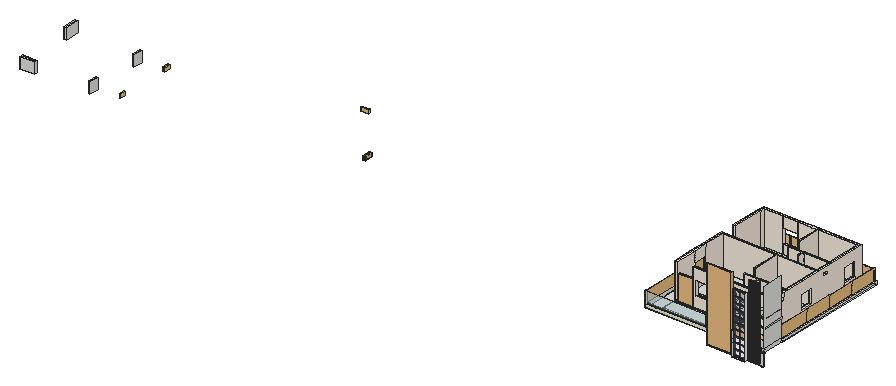
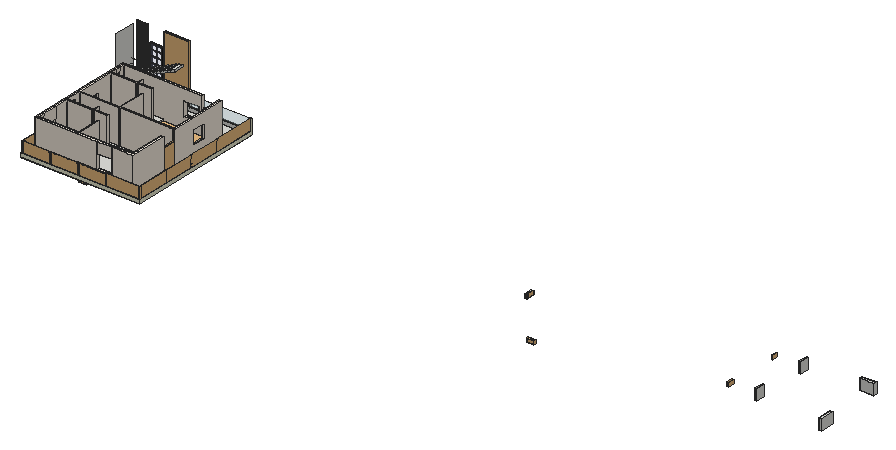
# SketchUp Ruby script. Lengths in inches.
U = 1.inch
M = Sketchup.active_model
def pt(a) = Geom::Point3d.new(a.map { |v| v * U })
def face(e, loops, mat)
  f = e.add_face(loops[0].map { |a| pt(a) })
  loops[1..].each { |l| e.add_face(l.map { |a| pt(a) }).erase! }
  f.material = f.back_material = mat if mat
  f
end
# faces: each face lists its corners as indices into pts; further lists are holes
def faces(e, pts, list, mat = nil) = list.each { |f| face(e, (f[0].is_a?(Array) ? f : [f]).map { |l| l.map { |i| pts[i] } }, mat) }
# xy, xz, yz: faces in a plane at the given z, y or x. An outline is a flat list of corners, or four numbers for a rectangle; further outlines are holes
def ring(l) = l.size == 4 ? [[l[0], l[1]], [l[2], l[1]], [l[2], l[3]], [l[0], l[3]]] : l.each_slice(2).to_a
def flat(e, list, mat, &to3) = list.each { |f| face(e, (f[0].is_a?(Array) ? f : [f]).map { |l| ring(l).map { |u, v| to3.(u, v) } }, mat) }
def xy(e, z, list, mat = nil) = flat(e, list, mat) { |x, y| [x, y, z] }
def xz(e, y, list, mat = nil) = flat(e, list, mat) { |x, z| [x, y, z] }
def yz(e, x, list, mat = nil) = flat(e, list, mat) { |y, z| [x, y, z] }
def lines(e, pts, list) = list.each { |a, b| e.add_line(pt(pts[a]), pt(pts[b])) }
# prism: a flat outline (further loops are holes) pulled along v
def prism(e, loops, v, mat = nil)
  f = face(e, loops, mat); d = Geom::Vector3d.new(v.map { |x| x * U })
  f.pushpull(f.normal.samedirection?(d) ? d.length : -d.length)
end
def box(e, o, s, mat = nil) = prism(e, [[o, [o[0] + s[0], o[1], o[2]], [o[0] + s[0], o[1] + s[1], o[2]], [o[0], o[1] + s[1], o[2]]]], [0, 0, s[2]], mat)
def at(x, y, z, deg = 0) = Geom::Transformation.translation(pt([x, y, z])) * Geom::Transformation.rotation(ORIGIN, Z_AXIS, deg.degrees)
def axes(o, x, y, z) = Geom::Transformation.new([*x, 0, *y, 0, *z, 0, *pt(o).to_a, 1])
def part(name) = M.definitions.add(name)
# library, detail: a bought-in or finely detailed component or shape, given as its bounding box
def library(name, o, s) = part(name).tap { |d| box(d.entities, o, s) }
def detail(e, o, s) = box(e.add_group.entities, o, s)
def put(e, d, t, mat = nil) = e.add_instance(d, t).tap { |i| i.material = mat if mat }
def group(e, t, mat = nil) = e.add_group.tap { |g| g.transformation = t; g.material = mat if mat }.entities
root = M.entities
M.materials.add("0037 AP 8028 PEACH ORGANZA").color = [246, 236, 223]
M.materials.add("0113 AP L161 ABSOLUTE WHITE").color = [243, 242, 236]
M.materials.add("0746 AP 7715 LUMINOUS").color = [235, 235, 209]
M.materials.add("Glass_Safety_01").color = [204, 235, 244]
M.materials["Glass_Safety_01"].alpha = 0.25
M.materials.add("Glass_Sky Reflection_01").color = [126, 138, 183]
M.materials["Glass_Sky Reflection_01"].alpha = 0.25
M.materials.add("M08_Obsidian_Black").color = [30, 30, 30]
M.materials.add("[0132_LightGray]").color = [169, 169, 169]
M.materials.add("[Metal Seamed]").color = [118, 119, 114]
c1 = library("Group\#46",[0,-3,0],[81.91,6,241.7])
c2 = library("Group\#25",[0,-0.05,0],[30,2.55,24])
c3 = part("Group19\#1")
p = [[1706.5625,247.76,0],[1706.5625,271.76,0],[1706.5625,427.76,65],[1706.5625,431.76,65],[1720.5625,431.76,65],[1720.5625,427.76,65],
  [1686.5625,247.76,0],[1686.5625,271.76,0],[1686.5625,427.76,65],[1686.5625,451.76,65],[1740.5625,451.76,65],[1740.5625,427.76,65]]
lines(c3.entities,p,[[0,1],[1,2],[2,3],[3,4],[4,5],[6,7],[7,8],[8,9],[9,10],[10,11]])
c4 = part("Group18\#2")
xy(c4.entities,-3.9375,[[1682.5625,269.14,1710.5625,281.14],[1684.29,281.14,1710.5625,281.93]])
xy(c4.entities,0,[[1682.5625,269.14,1710.5625,281.14]])
xy(c4.entities,5,[[1684.29,281.14,1710.5625,293.14]])
xy(c4.entities,10,[[1684.29,293.14,1710.5625,305.14]])
xy(c4.entities,15,[[1684.29,305.14,1710.5625,317.14]])
xy(c4.entities,20,[[1684.29,317.14,1710.5625,329.14]])
xy(c4.entities,25,[[1684.29,329.14,1710.5625,341.14]])
xy(c4.entities,30,[[1684.29,341.14,1710.5625,353.14]])
xy(c4.entities,35,[[1684.29,353.14,1710.5625,365.14]])
xy(c4.entities,40,[[1684.29,365.14,1710.5625,377.14]])
xy(c4.entities,45,[[1684.29,377.14,1710.5625,389.14]])
xy(c4.entities,50,[[1684.29,389.14,1710.5625,401.14]])
xy(c4.entities,55,[[1684.29,401.14,1710.5625,413.14]])
xy(c4.entities,60,[[1684.29,413.14,1710.5625,425.14]])
xy(c4.entities,61.0625,[[1716.5625,412.36,1744.5625,453.14],[1710.5625,425.14,1710.5625,437.93,1684.29,437.93,1684.29,453.14,1716.5625,453.14,1716.5625,425.14]])
xy(c4.entities,65,[[1716.5625,413.14,1744.5625,453.14],[1684.29,425.14,1716.5625,453.14]])
xy(c4.entities,70,[[1716.5625,401.14,1744.5625,413.14]])
xy(c4.entities,75,[[1716.5625,389.14,1744.5625,401.14]])
xy(c4.entities,80,[[1716.5625,377.14,1744.5625,389.14]])
xy(c4.entities,85,[[1716.5625,365.14,1744.5625,377.14]])
xy(c4.entities,90,[[1716.5625,353.14,1744.5625,365.14]])
xy(c4.entities,95,[[1716.5625,341.14,1744.5625,353.14]])
xy(c4.entities,100,[[1716.5625,329.14,1744.5625,341.14]])
xy(c4.entities,105,[[1716.5625,317.14,1744.5625,329.14]])
xy(c4.entities,110,[[1716.5625,305.14,1744.5625,317.14]])
xy(c4.entities,115,[[1716.5625,293.14,1744.5625,305.14]])
xy(c4.entities,120.6,[[1716.5625,281.14,1744.5625,293.14]])
xz(c4.entities,269.14,[[1682.5625,-3.9375,1710.5625,0]])
xz(c4.entities,281.14,[[1682.5625,-3.9375,1684.29,0],[1684.29,-3.9375,1710.5625,0],[1684.29,0,1710.5625,5],[1716.5625,115.73,1744.5625,120.6]])
xz(c4.entities,293.14,[[1684.29,5,1710.5625,10],[1716.5625,115,1744.5625,120.6]])
xz(c4.entities,305.14,[[1684.29,10,1710.5625,15],[1716.5625,110,1744.5625,115]])
xz(c4.entities,317.14,[[1684.29,15,1710.5625,20],[1716.5625,105,1744.5625,110]])
xz(c4.entities,329.14,[[1684.29,20,1710.5625,25],[1716.5625,100,1744.5625,105]])
xz(c4.entities,341.14,[[1684.29,25,1710.5625,30],[1716.5625,95,1744.5625,100]])
xz(c4.entities,353.14,[[1684.29,30,1710.5625,35],[1716.5625,90,1744.5625,95]])
xz(c4.entities,365.14,[[1684.29,35,1710.5625,40],[1716.5625,85,1744.5625,90]])
xz(c4.entities,377.14,[[1684.29,40,1710.5625,45],[1716.5625,80,1744.5625,85]])
xz(c4.entities,389.14,[[1684.29,45,1710.5625,50],[1716.5625,75,1744.5625,80]])
xz(c4.entities,401.14,[[1684.29,50,1710.5625,55],[1716.5625,70,1744.5625,75]])
xz(c4.entities,413.14,[[1684.29,55,1710.5625,60],[1716.5625,65,1744.5625,70]])
xz(c4.entities,425.14,[[1684.29,60,1710.5625,65],[1710.5625,61.0625,1716.5625,65]])
xz(c4.entities,453.14,[[1684.29,61.0625,1716.5625,65],[1716.5625,61.0625,1744.5625,65]])
yz(c4.entities,1682.5625,[[269.14,-3.9375,281.14,0]])
yz(c4.entities,1684.29,[[281.14,-3.9375,281.14,5,293.14,5,293.14,10,305.14,10,305.14,15,317.14,15,317.14,20,329.14,20,329.14,25,341.14,25,341.14,30,353.14,30,353.14,35,365.14,35,365.14,40,377.14,40,377.14,45,389.14,45,389.14,50,401.14,50,401.14,55,413.14,55,413.14,60,425.14,60,425.14,65,453.14,65,453.14,61.0625,437.93,61.0625,281.93,-3.9375]])
yz(c4.entities,1710.5625,[[269.14,-3.9375,281.14,0],[281.14,-3.9375,281.93,-3.9375,437.93,61.0625,425.14,61.0625,425.14,60,413.14,60,413.14,55,401.14,55,401.14,50,389.14,50,389.14,45,377.14,45,377.14,40,365.14,40,365.14,35,353.14,35,353.14,30,341.14,30,341.14,25,329.14,25,329.14,20,317.14,20,317.14,15,305.14,15,305.14,10,293.14,10,293.14,5,281.14,5]])
yz(c4.entities,1716.5625,[[412.36,61.0625,281.42,115.62,281.14,115.73,281.14,120.6,293.14,120.6,293.14,115,305.14,115,305.14,110,317.14,110,317.14,105,329.14,105,329.14,100,341.14,100,341.14,95,353.14,95,353.14,90,365.14,90,365.14,85,377.14,85,377.14,80,389.14,80,389.14,75,401.14,75,401.14,70,413.14,70,413.14,65,425.14,65,425.14,61.0625],[425.14,61.0625,453.14,65]])
yz(c4.entities,1744.5625,[[412.36,61.0625,453.14,61.0625,453.14,65,413.14,65,413.14,70,401.14,70,401.14,75,389.14,75,389.14,80,377.14,80,377.14,85,365.14,85,365.14,90,353.14,90,353.14,95,341.14,95,341.14,100,329.14,100,329.14,105,317.14,105,317.14,110,305.14,110,305.14,115,293.14,115,293.14,120.6,281.14,120.6,281.14,115.73]])
p = [[1710.5625,281.93,-3.9375],[1684.29,281.93,-3.9375],[1684.29,437.93,61.0625],[1710.5625,437.93,61.0625],[1744.5625,412.36,61.0625],[1744.5625,281.14,115.73],
  [1716.5625,281.42,115.62],[1716.5625,412.36,61.0625],[1716.5625,281.14,115.73]]
faces(c4.entities,p,[[0,1,2,3],[4,5,6,7],[8,6,5]])
put(c4.entities,c3,at(0,0,24))
c5 = library("Group\#2",[41.39,24.57,0],[327.06,423.03,0.01])
c6 = library("Group\#12",[0,0,0],[6.9375,42,86.5])
c7 = part("Group\#29")
xy(c7.entities,0,[[0,0,0,179.49,176.02,179.49,176.02,89,180.99,89,180.99,179.49,311,179.49,311,53,176.02,53,176.02,47.99,222,47.99,222,30.01,227.01,30.01,227.01,47.99,311,47.99,311,0]])
c8 = library("skp9290",[5.02,1.95,0],[10.03,3.89,0.08])
box(root,[272,323.41,84],[5.01,30,36])
box(root,[272,138.91,84],[5.01,30,36])
box(root,[50,129.92,84],[48.03,8.99,36])
box(root,[41.01,323.41,84],[8.99,47.98,36])
xy(root,73.55,[[2370.2,117.37,2549.9,117.53]])
xy(root,73.55,[[2452.6,108.36,2495.6,117.37]],"0113 AP L161 ABSOLUTE WHITE")
xy(root,80.8,[[2370.2,103.36,2448.6,112.36],[2506.22,109.7,2507.72,110.7],[2511.22,109.7,2512.72,110.7],[2516.22,109.7,2517.72,110.7],[2521.22,109.7,2522.72,110.7],
  [2526.22,109.7,2527.72,110.7],[2531.22,109.7,2532.72,110.7],[2536.22,109.7,2537.72,110.7],[2541.22,109.7,2542.72,110.7],[2366.69,112.36,2370.2,117.37]])
xy(root,92.44,[[2519.38,354.52,2528.37,379.54]])
xy(root,96,[[1066.63,294.4,1075.625,319.41]])
xy(root,104.08,[[2519.38,354.52,2528.37,379.54]])
xy(root,108,[[1066.63,294.4,1075.625,319.41]])
xy(root,115.5,[[2155.9,112.36,2160.9,117.37],[2160.9,112.36,2366.69,117.37],[2549.9,112.36,2550.375,117.37],[2155.9,117.37,2160.9,579.4],[2549.9,117.37,2550.375,117.53],
  [2525.88,189.89,2549.9,192.78],[2549.9,192.78,2554.91,584.4],[2155.9,579.4,2549.9,584.4]])
xy(root,127.5,[[2160.9,112.36,2366.69,112.36,2366.69,117.37,2160.9,117.37,2160.9,115.67,2361.69,115.67,2361.69,113.67,2160.9,113.67],[2160.9,113.67,2361.69,115.67],[2155.9,117.37,2160.9,579.4],[2549.9,189.89,2554.91,584.4],[2155.9,579.4,2549.9,584.4]])
xz(root,109.7,[[2506.22,80.8,2507.72,322.5],[2511.22,80.8,2512.72,322.5],[2516.22,80.8,2517.72,322.5],[2521.22,80.8,2522.72,322.5],[2526.22,80.8,2527.72,322.5],
  [2531.22,80.8,2532.72,322.5],[2536.22,80.8,2537.72,322.5],[2541.22,80.8,2542.72,322.5]],"[0132_LightGray]")
xz(root,110.7,[[2506.22,80.8,2507.72,322.5],[2511.22,80.8,2512.72,322.5],[2516.22,80.8,2517.72,322.5],[2521.22,80.8,2522.72,322.5],[2526.22,80.8,2527.72,322.5],
  [2531.22,80.8,2532.72,322.5],[2536.22,80.8,2537.72,322.5],[2541.22,80.8,2542.72,322.5]])
xz(root,112.36,[[2155.9,115.5,2366.69,115.5,2366.69,127.5,2160.9,127.5,2160.9,164.58,2155.9,164.58]],"0746 AP 7715 LUMINOUS")
xz(root,113.67,[[2160.9,127.5,2361.69,164.58]],"Glass_Safety_01")
xz(root,115.67,[[2160.9,127.5,2361.69,164.58]],"Glass_Safety_01")
xz(root,117.37,[[2370.2,73.55,2452.6,115.5],[2495.6,73.55,2549.9,115.5],[2366.69,80.8,2370.2,115.5],[2160.9,115.5,2452.6,127.5],[2495.6,115.5,2549.9,127.5],
  [2366.69,127.5,2452.6,151.5],[2495.6,127.5,2549.9,151.5]])
xz(root,117.37,[[2155.9,127.5,2160.9,164.58]],"0746 AP 7715 LUMINOUS")
xz(root,294.4,[[1066.63,96,1075.625,108]])
xz(root,319.41,[[1066.63,96,1075.625,108]])
xz(root,354.52,[[2519.38,92.44,2528.37,104.08]])
xz(root,379.54,[[2519.38,92.44,2528.37,104.08]])
xz(root,579.4,[[2160.9,115.5,2549.9,127.5]])
xz(root,584.4,[[2155.9,115.5,2554.91,127.5]],"0746 AP 7715 LUMINOUS")
yz(root,2155.9,[[112.36,115.5,112.36,164.58,117.37,164.58,117.37,127.5,584.4,127.5,584.4,115.5]],"0746 AP 7715 LUMINOUS")
yz(root,2160.9,[[117.37,115.5,579.4,127.5],[112.36,127.5,113.67,164.58],[113.67,127.5,115.67,164.58],[115.67,127.5,117.37,164.58]])
yz(root,2361.69,[[113.67,127.5,115.67,164.58]])
yz(root,2366.69,[[112.36,127.5,117.37,151.5]])
yz(root,2366.69,[[112.36,80.8,117.37,115.5]],"0746 AP 7715 LUMINOUS")
yz(root,2448.6,[[108.36,80.8,112.36,151.5]])
yz(root,2452.6,[[108.36,115.5,117.37,127.5],[108.36,127.5,117.37,151.49]])
yz(root,2452.6,[[108.36,73.55,117.37,115.5]],"0113 AP L161 ABSOLUTE WHITE")
yz(root,2495.6,[[108.36,73.55,117.37,274.5]],"0113 AP L161 ABSOLUTE WHITE")
yz(root,2506.22,[[109.7,80.8,110.7,322.5]],"[0132_LightGray]")
yz(root,2507.72,[[109.7,80.8,110.7,322.5]],"[0132_LightGray]")
yz(root,2511.22,[[109.7,80.8,110.7,322.5]],"[0132_LightGray]")
yz(root,2512.72,[[109.7,80.8,110.7,322.5]],"[0132_LightGray]")
yz(root,2516.22,[[109.7,80.8,110.7,322.5]],"[0132_LightGray]")
yz(root,2517.72,[[109.7,80.8,110.7,322.5]],"[0132_LightGray]")
yz(root,2521.22,[[109.7,80.8,110.7,322.5]],"[0132_LightGray]")
yz(root,2522.72,[[109.7,80.8,110.7,322.5]],"[0132_LightGray]")
yz(root,2525.88,[[189.89,115.5,192.78,235.5]])
yz(root,2526.22,[[109.7,80.8,110.7,322.5]],"[0132_LightGray]")
yz(root,2527.72,[[109.7,80.8,110.7,322.5]],"[0132_LightGray]")
yz(root,2531.22,[[109.7,80.8,110.7,322.5]],"[0132_LightGray]")
yz(root,2532.72,[[109.7,80.8,110.7,322.5]],"[0132_LightGray]")
yz(root,2536.22,[[109.7,80.8,110.7,322.5]],"[0132_LightGray]")
yz(root,2537.72,[[109.7,80.8,110.7,322.5]],"[0132_LightGray]")
yz(root,2541.22,[[109.7,80.8,110.7,322.5]],"[0132_LightGray]")
yz(root,2542.72,[[109.7,80.8,110.7,322.5]],"[0132_LightGray]")
yz(root,2549.9,[[117.37,73.55,117.53,115.5],[112.36,115.5,117.37,127.5],[117.37,115.5,579.4,127.5],[117.37,127.5,189.89,313.5]])
p = [[2528.375,194.04,120],[2554.91,194.04,120],[2554.91,112.36,120],[2550.375,112.36,120],[2550.375,191.07,120],[2554.91,191.07,120],
  [2554.91,189.89,115.5],[2549.9,189.89,115.5],[2549.9,117.37,127.5],[2554.91,117.37,127.5],[2550.375,112.36,115.5],[2554.91,112.36,115.5],
  [2550.375,117.37,115.5],[2554.91,117.37,115.5],[2370.2,112.36,115.5],[2370.2,117.37,115.5]]
lines(root,p,[[0,1],[2,3],[4,5],[6,7],[8,9],[10,11],[12,13],[14,15]])
g1 = group(root,at(2452.6,117.3,73.55),"M08_Obsidian_Black")
xy(g1,0,[[42.95,-4.93,-0.06,-4.2,0,0.73,43,0]])
xy(g1,0.8,[[41.96,-4.91,41.97,-3.72,21.66,-3.37,21.46,-3.37,0.94,-3.02,0.93,-4.22],[41.97,-3.72,42.01,0.02,0.99,0.71,0.94,-3.02,21.46,-3.37,21.66,-3.37]])
xy(g1,200.15,[[41.96,-4.91,0.93,-4.22,0.94,-3.02,21.46,-3.37,21.66,-3.37,41.97,-3.72],[41.97,-3.72,21.66,-3.37,21.46,-3.37,0.94,-3.02,0.99,0.71,42.01,0.02]])
xy(g1,200.95,[[42.95,-4.93,43,0,0,0.73,-0.06,-4.2]])
xz(g1,-3.37,[[21.46,0.8,21.66,200.15]],"M08_Obsidian_Black")
p = [[42.95,-4.93,200.95],[-0.06,-4.2,200.95],[-0.06,-4.2,0],[42.95,-4.93,0],[41.96,-4.91,0.8],[0.93,-4.22,0.8],
  [0.93,-4.22,200.15],[41.96,-4.91,200.15],[43,0,0],[43,0,200.95],[0,0.73,200.95],[0,0.73,0],
  [0.99,0.71,0.8],[42.01,0.02,0.8],[42.01,0.02,200.15],[0.99,0.71,200.15],[41.97,-3.72,200.15],[41.97,-3.72,199.98],
  [41.97,-3.72,180.28],[41.97,-3.72,180.11],[41.97,-3.72,160.41],[41.97,-3.72,160.24],[41.97,-3.72,140.54],[41.97,-3.72,140.37],
  [41.97,-3.72,120.67],[41.97,-3.72,120.5],[41.97,-3.72,100.8],[41.97,-3.72,100.63],[41.97,-3.72,80.93],[41.97,-3.72,80.76],
  [41.97,-3.72,61.06],[41.97,-3.72,60.89],[41.97,-3.72,41.19],[41.97,-3.72,41.02],[41.97,-3.72,21.32],[41.97,-3.72,21.15],
  [41.97,-3.72,1.45],[41.97,-3.72,1.28],[41.97,-3.72,0.8],[0.94,-3.02,0.8],[0.94,-3.02,1.28],[0.94,-3.02,1.45],
  [0.94,-3.02,21.15],[0.94,-3.02,21.32],[0.94,-3.02,41.02],[0.94,-3.02,41.19],[0.94,-3.02,60.89],[0.94,-3.02,61.06],
  [0.94,-3.02,80.76],[0.94,-3.02,80.93],[0.94,-3.02,100.63],[0.94,-3.02,100.8],[0.94,-3.02,120.5],[0.94,-3.02,120.67],
  [0.94,-3.02,140.37],[0.94,-3.02,140.54],[0.94,-3.02,160.24],[0.94,-3.02,160.41],[0.94,-3.02,180.11],[0.94,-3.02,180.28],
  [0.94,-3.02,199.98],[0.94,-3.02,200.15],[21.66,-3.37,1.28],[21.66,-3.37,0.8],[21.46,-3.37,0.8],[21.46,-3.37,1.28],
  [21.66,-3.37,1.45],[21.46,-3.37,1.45],[21.66,-3.37,21.15],[21.46,-3.37,21.15],[21.66,-3.37,21.32],[21.46,-3.37,21.32],
  [21.66,-3.37,41.02],[21.46,-3.37,41.02],[21.66,-3.37,41.19],[21.46,-3.37,41.19],[21.66,-3.37,60.89],[21.46,-3.37,60.89],
  [21.66,-3.37,61.06],[21.46,-3.37,61.06],[21.66,-3.37,80.76],[21.46,-3.37,80.76],[21.66,-3.37,80.93],[21.46,-3.37,80.93],
  [21.66,-3.37,100.63],[21.46,-3.37,100.63],[21.66,-3.37,100.8],[21.46,-3.37,100.8],[21.66,-3.37,120.5],[21.46,-3.37,120.5],
  [21.66,-3.37,120.67],[21.46,-3.37,120.67],[21.66,-3.37,140.37],[21.46,-3.37,140.37],[21.66,-3.37,140.54],[21.46,-3.37,140.54],
  [21.66,-3.37,160.24],[21.46,-3.37,160.24],[21.66,-3.37,160.41],[21.46,-3.37,160.41],[21.66,-3.37,180.11],[21.46,-3.37,180.11],
  [21.66,-3.37,180.28],[21.46,-3.37,180.28],[21.66,-3.37,199.98],[21.46,-3.37,199.98],[21.66,-3.37,200.15],[21.46,-3.37,200.15]]
faces(g1,p,[[[0,1,2,3],[4,5,6,7]],[66,62,37,36],[65,67,41,40],[70,68,35,34],[69,71,43,42],[74,72,33,32],[73,75,45,44],[78,76,31,30],
  [77,79,47,46],[82,80,29,28],[81,83,49,48],[86,84,27,26],[85,87,51,50],[90,88,25,24],[89,91,53,52],[94,92,23,22],
  [93,95,55,54],[98,96,21,20],[97,99,57,56],[102,100,19,18],[101,103,59,58],[106,104,17,16],[61,60,105,107]],"M08_Obsidian_Black")
faces(g1,p,[[8,9,0,3],[10,11,2,1],[[10,9,8,11],[12,13,14,15]],[7,16,17,18,19,20,21,22,23,24,25,26,27,28,29,30,31,32,33,34,35,36,37,38,4],[5,39,40,41,42,43,44,45,46,47,48,49,50,51,52,53,54,55,56,57,58,59,60,61,6],[14,13,38,37,36,35,34,33,32,31,30,29,28,27,26,25,24,23,22,21,20,19,18,17,16],[12,15,61,60,59,58,57,56,55,54,53,52,51,50,49,48,47,46,45,44,43,42,41,40,39]])
faces(g1,p,[[38,37,62,63],[64,65,40,39],[68,66,36,35],[42,41,67,69],[72,70,34,33],[44,43,71,73],[76,74,32,31],[46,45,75,77],
  [80,78,30,29],[48,47,79,81],[84,82,28,27],[50,49,83,85],[88,86,26,25],[52,51,87,89],[92,90,24,23],[54,53,91,93],
  [96,94,22,21],[56,55,95,97],[100,98,20,19],[58,57,99,101],[104,102,18,17],[60,59,103,105]],"Glass_Sky Reflection_01")
put(root,c1,at(2366.69,112.36,80.8))
put(root,c2,axes([2354.36,553.61,92.44],[0.8,0,0],[0,1.82683,0],[0,0,0.485]))
put(root,c2,axes([2521.38,379.54,92.44],[0,-0.83382,0],[1.82683,0,0],[0,0,0.485]))
put(root,c2,axes([363,171.91,95.92],[0,-0.60073,0],[1.82683,0,0],[0,0,0.50315]))
put(root,c2,axes([363,357.39,95.92],[0,-0.66205,0],[1.82683,0,0],[0,0,0.51171]))
put(root,c2,axes([901.62,493.49,96],[0.8,0,0],[0,1.82683,0],[0,0,0.5]))
put(root,c2,axes([1068.63,319.41,96],[0,-0.83382,0],[1.82683,0,0],[0,0,0.5]))
put(root,c4,axes([2084.98,2150.13,119.72],[0.0107,-1.16479,0],[0.99132,0.00911,0],[0,0,1.07141]))
g2 = group(root,at(2160.9,560.39,115.5))
xy(g2,0,[[0,-443.02,36,-370.5],[36,-443.02,209.22,-370.5],[0,-370.5,36,0],[209.22,-370.5,364.98,-367.61],[364.98,-367.61,388.99,0],
  [0,0,364.98,19.01],[364.98,0,388.99,19.01]])
xy(g2,1,[[0,-443.02,209.22,-443.02,209.22,-370.5,36,-370.5,36,0,364.98,0,364.98,19.01,0,19.01],[209.22,-370.5,364.98,-367.61],[364.98,-367.61,388.99,0],[364.98,0,388.99,19.01]])
xz(g2,-443.02,[[0,0,36,1],[36,0,209.22,1]])
xz(g2,-370.5,[[36,0,364.98,1]])
xz(g2,-367.61,[[209.22,0,388.99,1]])
xz(g2,0,[[36,0,364.98,1],[364.98,0,388.99,1]])
xz(g2,19.01,[[0,0,364.98,1],[364.98,0,388.99,1]])
yz(g2,0,[[-443.02,0,-370.5,1],[-370.5,0,0,1],[0,0,19.01,1]])
yz(g2,36,[[-370.5,0,0,1]])
yz(g2,209.22,[[-443.02,0,-367.61,1]])
yz(g2,364.98,[[-370.5,0,0,1],[0,0,19.01,1]])
yz(g2,388.99,[[-367.61,0,0,1],[0,0,19.01,1]])
put(root,c5,at(2155.9,112.36,115.5))
put(root,c6,axes([2426.9,383.38,115.5],[0.86547,0,0],[0,0.71448,0],[0,0,0.9711]))
put(root,c6,axes([2253.93,190.32,115.5],[0,0.89531,0],[-1.14256,0,0],[0,0,0.9711]))
g3 = group(root,at(2196.91,535.62,115.5),"0037 AP 8028 PEACH ORGANZA")
xy(g3,0,[[0,-345.73,8.99,-275.49],[57.02,-345.73,319.99,-336.74],[319.99,-345.73,328.98,-336.74],[319.99,-336.74,328.98,-321.76],[319.99,-321.76,328.98,-303.74],
  [230.99,-306.73,236,-288.76],[319.99,-303.74,328.98,-288.76],[185.01,-288.76,230.99,-283.75],[230.99,-288.76,236,-283.75],[236,-288.76,236.3,-283.75],
  [236.3,-288.76,319.99,-283.75],[319.99,-288.76,328.98,-283.75],[319.99,-283.75,328.98,-220.31],[0,-275.49,8.99,-227.5],[185.01,-247.75,189.98,-157.25],
  [0,-227.5,8.99,-157.25],[319.99,-220.31,328.98,-152.24],[0,-157.25,8.99,-152.24],[8.99,-157.25,185.01,-152.24],[185.01,-157.25,189.98,-152.24],
  [189.98,-157.25,319.99,-152.24],[319.99,-152.24,328.98,-104.25],[230.99,-122.23,236,-104.25],[0,-104.25,8.99,0],[185.01,-104.25,230.99,-99.25],
  [230.99,-104.25,236,-99.25],[236,-104.25,319.99,-99.25],[319.99,-104.25,328.98,-99.25],[319.99,-99.25,328.98,-51.73],[185.01,-63.24,189.98,15.78],
  [319.99,-51.73,328.98,-3.7],[319.99,-3.7,328.98,15.78],[0,0,8.99,15.78],[0,15.78,71.96,24.77],[71.96,15.78,119.95,24.77],
  [119.95,15.78,185.01,24.77],[185.01,15.78,189.98,24.77],[189.98,15.78,319.99,24.77],[319.99,15.78,328.98,24.77]])
xy(g3,1,[[8.99,-152.24,8.99,15.78,185.01,15.78,185.01,-63.24,189.98,-63.24,189.98,15.78,319.99,15.78,319.99,-99.25,185.01,-99.25,185.01,-104.25,230.99,-104.25,230.99,-122.23,236,-122.23,236,-104.25,319.99,-104.25,319.99,-152.24]])
xy(g3,36,[[319.99,-233.25,328.98,-185.25],[319.99,-51.73,328.98,-3.7],[71.96,15.78,119.95,24.77]])
xy(g3,37,[[0,-275.49,8.99,-227.5]])
xy(g3,37,[[69.02,-345.73,117.02,-336.74]],"0037 AP 8028 PEACH ORGANZA")
xy(g3,84,[[319.99,-233.25,328.98,-185.25],[319.99,-51.73,328.98,-3.7],[71.96,15.78,119.95,24.77]])
xy(g3,85,[[0,-275.49,8.99,-227.5]])
xy(g3,85,[[69.02,-345.73,117.02,-336.74]],"0037 AP 8028 PEACH ORGANZA")
xy(g3,95.92,[[319.99,-138.12,328.98,-118.25]])
xy(g3,96,[[319.99,-321.76,328.98,-303.74]])
xy(g3,108,[[319.99,-321.76,328.98,-303.74]])
xy(g3,108.21,[[319.99,-138.12,328.98,-118.25]])
xy(g3,120,[[0,-345.73,8.99,-275.49],[57.02,-345.73,319.99,-336.74],[319.99,-345.73,328.98,-336.74],[319.99,-336.74,328.98,-321.76],[319.99,-321.76,328.98,-303.74],
  [230.99,-306.73,236,-288.76],[319.99,-303.74,328.98,-288.76],[185.01,-288.76,230.99,-283.75],[230.99,-288.76,236,-283.75],[236,-288.76,236.3,-283.75],
  [236.3,-288.76,319.99,-283.75],[319.99,-288.76,328.98,-283.75],[319.99,-283.75,328.98,-220.31],[0,-275.49,8.99,-227.5],[185.01,-247.75,189.98,-157.25],
  [0,-227.5,8.99,-157.25],[319.99,-220.31,328.98,-152.24],[0,-157.25,8.99,-152.24],[8.99,-157.25,185.01,-152.24],[185.01,-157.25,189.98,-152.24],
  [189.98,-157.25,319.99,-152.24],[319.99,-152.24,328.98,-104.25],[230.99,-122.23,236,-104.25],[0,-104.25,8.99,0],[185.01,-104.25,230.99,-99.25],
  [230.99,-104.25,236,-99.25],[236,-104.25,319.99,-99.25],[319.99,-104.25,328.98,-99.25],[319.99,-99.25,328.98,-51.73],[185.01,-63.24,189.98,15.78],
  [319.99,-51.73,328.98,-3.7],[319.99,-3.7,328.98,15.78],[0,0,8.99,15.78],[0,15.78,71.96,24.77],[71.96,15.78,119.95,24.77],
  [119.95,15.78,185.01,24.77],[185.01,15.78,189.98,24.77],[189.98,15.78,319.99,24.77],[319.99,15.78,328.98,24.77]])
xz(g3,-345.73,[[0,0,8.99,120],[319.99,0,328.98,120]])
xz(g3,-345.73,[[[57.02,0,319.99,120],[69.02,37,117.02,85]]],"0037 AP 8028 PEACH ORGANZA")
xz(g3,-336.74,[[[57.02,0,319.99,120],[69.02,37,117.02,85]]])
xz(g3,-321.76,[[319.99,96,328.98,108],[319.99,108,328.98,120]])
xz(g3,-306.73,[[230.99,0,236,120]])
xz(g3,-303.74,[[319.99,96,328.98,108],[319.99,108,328.98,120]])
xz(g3,-288.76,[[185.01,0,230.99,120],[230.99,0,236,120],[236,0,236.3,120],[236.3,0,319.99,120]])
xz(g3,-283.75,[[185.01,0,230.99,120],[230.99,0,236,120],[236,0,236.3,120],[236.3,0,319.99,120]])
xz(g3,-275.49,[[0,37,8.99,85]])
xz(g3,-247.75,[[185.01,0,189.98,120]])
xz(g3,-233.25,[[319.99,36,328.98,84]])
xz(g3,-227.5,[[0,37,8.99,85]])
xz(g3,-185.25,[[319.99,36,328.98,84]])
xz(g3,-157.25,[[8.99,0,185.01,120],[185.01,0,189.98,120],[189.98,0,319.99,120]])
xz(g3,-152.24,[[0,0,8.99,120],[8.99,0,185.01,1],[185.01,0,189.98,1],[189.98,0,319.99,1],[8.99,1,185.01,120],
  [185.01,1,189.98,120],[189.98,1,319.99,120]])
xz(g3,-138.12,[[319.99,95.92,328.98,108.21]])
xz(g3,-122.23,[[230.99,0,236,1],[230.99,1,236,120]])
xz(g3,-118.25,[[319.99,95.92,328.98,108.21]])
xz(g3,-104.25,[[0,0,8.99,120],[185.01,0,230.99,1],[230.99,0,236,120],[236,0,319.99,1],[185.01,1,230.99,120],
  [236,1,319.99,120]])
xz(g3,-99.25,[[185.01,0,230.99,1],[230.99,0,236,1],[236,0,319.99,1],[185.01,1,230.99,120],[230.99,1,236,120],
  [236,1,319.99,120]])
xz(g3,-63.24,[[185.01,0,189.98,1],[185.01,1,189.98,120]])
xz(g3,-51.73,[[319.99,0,328.98,36],[319.99,36,328.98,84]])
xz(g3,-3.7,[[319.99,0,328.98,36],[319.99,36,328.98,84]])
xz(g3,15.78,[[8.99,0,71.96,1],[71.96,0,119.95,1],[119.95,0,185.01,1],[185.01,0,189.98,120],[189.98,0,319.99,1],
  [8.99,1,71.96,120],[71.96,1,119.95,36],[119.95,1,185.01,120],[189.98,1,319.99,120],[71.96,84,119.95,120]])
xz(g3,24.77,[[0,0,71.96,120],[71.96,0,119.95,36],[119.95,0,328.98,120],[71.96,84,119.95,120]])
yz(g3,0,[[[-345.73,0,-152.24,120],[-275.49,37,-227.5,85]],[-104.25,0,24.77,120]])
yz(g3,8.99,[[-345.73,0,-275.49,120],[-275.49,0,-227.5,37],[-227.5,0,-157.25,120],[-157.25,0,-152.24,120],[-152.24,0,-104.25,1],
  [-104.25,0,0,1],[0,0,15.78,1],[-104.25,1,0,120],[0,1,15.78,120],[-275.49,85,-227.5,120]])
yz(g3,57.02,[[-345.73,0,-336.74,120]])
yz(g3,69.02,[[-345.73,37,-336.74,85]],"0037 AP 8028 PEACH ORGANZA")
yz(g3,71.96,[[15.78,0,24.77,36],[15.78,36,24.77,84],[15.78,84,24.77,120]])
yz(g3,117.02,[[-345.73,37,-336.74,85]],"0037 AP 8028 PEACH ORGANZA")
yz(g3,119.95,[[15.78,0,24.77,36],[15.78,36,24.77,84],[15.78,84,24.77,120]])
yz(g3,185.01,[[-288.76,0,-283.75,120],[-247.75,0,-157.25,120],[-157.25,0,-152.24,120],[-104.25,0,-99.25,1],[-63.24,0,15.78,1],
  [-104.25,1,-99.25,120],[-63.24,1,15.78,120]])
yz(g3,189.98,[[-247.75,0,-157.25,120],[-157.25,0,-152.24,120],[-63.24,0,15.78,1],[-63.24,1,15.78,120]])
yz(g3,230.99,[[-306.73,0,-288.76,120],[-288.76,0,-283.75,120],[-122.23,0,-104.25,1],[-104.25,0,-99.25,120],[-122.23,1,-104.25,120]])
yz(g3,236,[[-306.73,0,-288.76,120],[-288.76,0,-283.75,120],[-122.23,0,-104.25,1],[-104.25,0,-99.25,120],[-122.23,1,-104.25,120]])
yz(g3,236.3,[[-288.76,0,-283.75,120]])
yz(g3,319.99,[[-345.73,0,-336.74,120],[-336.74,0,-321.76,120],[-321.76,0,-303.74,96],[-303.74,0,-288.76,120],[-288.76,0,-283.75,120],
  [[-283.75,0,-157.25,120],[-233.25,36,-185.25,84]],[-157.25,0,-152.24,120],[-152.24,0,-104.25,1],[-104.25,0,-99.25,120],[-99.25,0,-51.73,1],
  [-51.73,0,-3.7,1],[-3.7,0,15.78,1],[[-152.24,1,-104.25,120],[-138.12,95.92,-118.25,108.21]],[-99.25,1,-51.73,120],[-51.73,1,-3.7,36],
  [-3.7,1,15.78,120],[-51.73,84,-3.7,120],[-321.76,108,-303.74,120]])
yz(g3,328.98,[[[-345.73,0,-220.31,0,-220.31,36,-233.25,36,-233.25,84,-185.25,84,-185.25,36,-220.31,36,-220.31,0,-51.73,0,-51.73,84,-3.7,84,-3.7,0,24.77,0,24.77,120,-303.74,120,-303.74,96,-321.76,96,-321.76,120,-345.73,120],[-138.12,95.92,-118.25,108.21]],[-51.73,0,-3.7,36],[-321.76,108,-303.74,120]])
put(g3,c7,at(8.99,-336.74,0))
put(root,c6,axes([2426.96,198.88,115.5],[0.85748,0,0],[0,0.71448,0],[0,0,0.9711]))
put(root,c6,axes([2197.32,383.38,115.5],[0.85622,0,0],[0,1.14256,0],[0,0,0.9711]))
g4 = group(root,at(2205.9,189.89,115.5))
box(g4,[0,0,0],[48.03,8.99,1])
g5 = group(root,at(2199.39,248.46,115.72))
xy(g5,0,[[0,0,0,312.08,328.98,312.08,328.98,0.06,184.97,0.06,184.97,0],[184.97,0,328.98,0.06]])
xy(g5,5.82,[[0,0,328.98,312.08]])
xz(g5,0,[[0,0,328.98,5.82]])
xz(g5,312.08,[[0,0,328.98,5.82]])
yz(g5,0,[[0,0,312.08,5.82]])
yz(g5,328.98,[[0,0,312.08,5.82]])
g6 = group(g5,at(184.97,-58.42,0))
box(g6,[0,0,0],[144,58.42,5.82])
put(root,c8,axes([2159.02,637,108.95],[0,-11.12631,0],[0,0,9.5202],[-14.2803,0,0]),"[Metal Seamed]")
put(root,c8,axes([2159.02,528.75,108.95],[0,-11.12631,0],[0,0,9.5202],[-14.2803,0,0]),"[Metal Seamed]")
put(root,c8,axes([2407.11,580.84,108.97],[9.5202,0,0],[0,0,9.5202],[0,-14.2803,0]),"[Metal Seamed]")
put(root,c8,axes([2314.48,580.84,108.97],[9.5202,0,0],[0,0,9.5202],[0,-14.2803,0]),"[Metal Seamed]")
put(root,c8,axes([2221.84,580.84,108.97],[9.5202,0,0],[0,0,9.5202],[0,-14.2803,0]),"[Metal Seamed]")
put(root,c8,axes([2098.05,580.84,108.97],[11.59093,0,0],[0,0,9.5202],[0,-14.2803,0]),"[Metal Seamed]")
put(root,c8,axes([2159.02,420.49,108.97],[0,-11.12631,0],[0,0,9.5202],[-14.2803,0,0]),"[Metal Seamed]")
put(root,c8,axes([2159.02,325.93,108.97],[0,-13.85767,0],[0,0,9.5202],[-14.2803,0,0]),"[Metal Seamed]")
g7 = group(root,at(2361.69,112.36,127.5),"0746 AP 7715 LUMINOUS")
box(g7,[0,0,0],[5,5,37.08])
put(root,c8,axes([2550.02,630,108.97],[0,-9.5202,0],[0,0,9.5202],[-14.2803,0,0]),"[Metal Seamed]")
put(root,c8,axes([2550.02,537.35,108.97],[0,-9.5202,0],[0,0,9.5202],[-14.2803,0,0]),"[Metal Seamed]")
put(root,c8,axes([2550.02,444.72,108.97],[0,-9.5202,0],[0,0,9.5202],[-14.2803,0,0]),"[Metal Seamed]")
put(root,c8,axes([2550.02,360.14,108.97],[0,-11.12631,0],[0,0,9.5202],[-14.2803,0,0]),"[Metal Seamed]")
